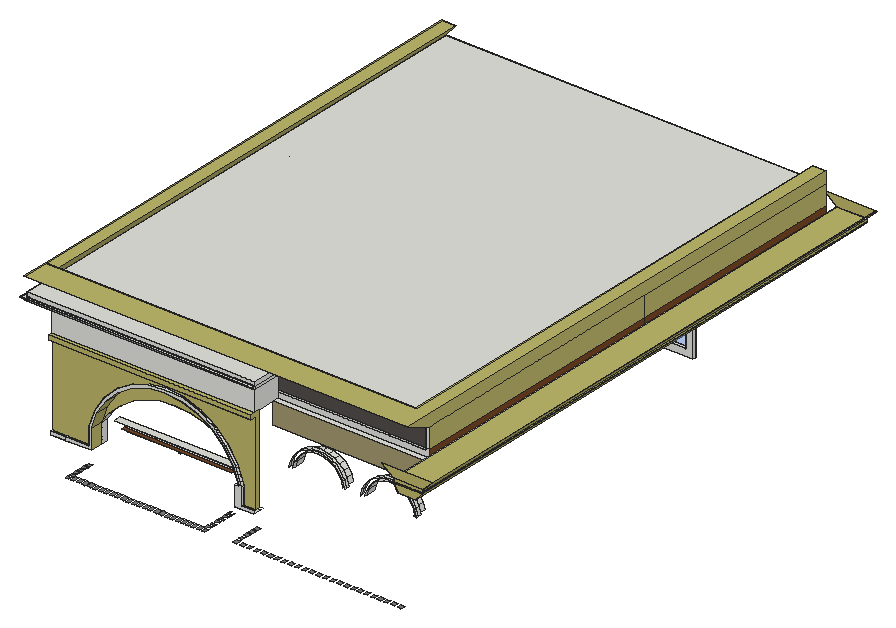
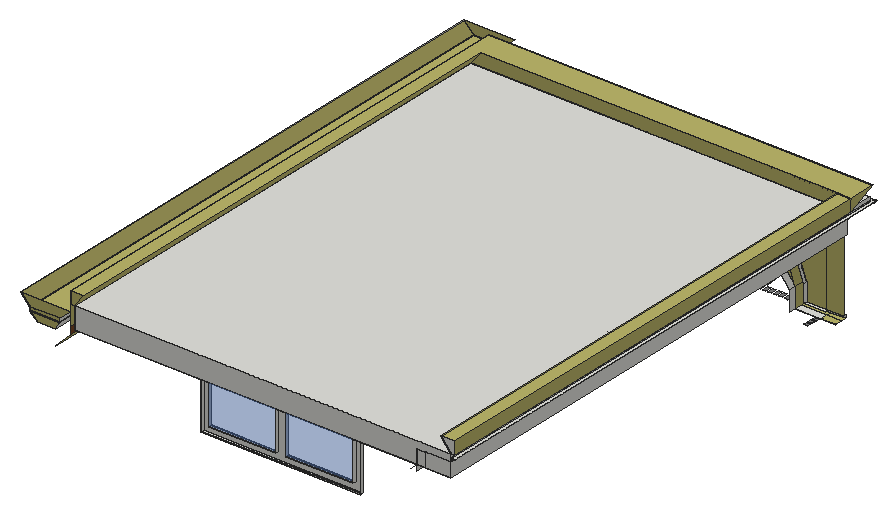
# SketchUp Ruby script. Lengths in inches.
U = 1.inch
M = Sketchup.active_model
def pt(a) = Geom::Point3d.new(a.map { |v| v * U })
def face(e, loops, mat)
  f = e.add_face(loops[0].map { |a| pt(a) })
  loops[1..].each { |l| e.add_face(l.map { |a| pt(a) }).erase! }
  f.material = f.back_material = mat if mat
  f
end
# faces: each face lists its corners as indices into pts; further lists are holes
def faces(e, pts, list, mat = nil) = list.each { |f| face(e, (f[0].is_a?(Array) ? f : [f]).map { |l| l.map { |i| pts[i] } }, mat) }
# xy, xz, yz: faces in a plane at the given z, y or x. An outline is a flat list of corners, or four numbers for a rectangle; further outlines are holes
def ring(l) = l.size == 4 ? [[l[0], l[1]], [l[2], l[1]], [l[2], l[3]], [l[0], l[3]]] : l.each_slice(2).to_a
def flat(e, list, mat, &to3) = list.each { |f| face(e, (f[0].is_a?(Array) ? f : [f]).map { |l| ring(l).map { |u, v| to3.(u, v) } }, mat) }
def xy(e, z, list, mat = nil) = flat(e, list, mat) { |x, y| [x, y, z] }
def xz(e, y, list, mat = nil) = flat(e, list, mat) { |x, z| [x, y, z] }
def yz(e, x, list, mat = nil) = flat(e, list, mat) { |y, z| [x, y, z] }
def lines(e, pts, list) = list.each { |a, b| e.add_line(pt(pts[a]), pt(pts[b])) }
# prism: a flat outline (further loops are holes) pulled along v
def prism(e, loops, v, mat = nil)
  f = face(e, loops, mat); d = Geom::Vector3d.new(v.map { |x| x * U })
  f.pushpull(f.normal.samedirection?(d) ? d.length : -d.length)
end
def box(e, o, s, mat = nil) = prism(e, [[o, [o[0] + s[0], o[1], o[2]], [o[0] + s[0], o[1] + s[1], o[2]], [o[0], o[1] + s[1], o[2]]]], [0, 0, s[2]], mat)
def at(x, y, z, deg = 0) = Geom::Transformation.translation(pt([x, y, z])) * Geom::Transformation.rotation(ORIGIN, Z_AXIS, deg.degrees)
def axes(o, x, y, z) = Geom::Transformation.new([*x, 0, *y, 0, *z, 0, *pt(o).to_a, 1])
def part(name) = M.definitions.add(name)
# library, detail: a bought-in or finely detailed component or shape, given as its bounding box
def library(name, o, s) = part(name).tap { |d| box(d.entities, o, s) }
def detail(e, o, s) = box(e.add_group.entities, o, s)
def put(e, d, t, mat = nil) = e.add_instance(d, t).tap { |i| i.material = mat if mat }
def group(e, t, mat = nil) = e.add_group.tap { |g| g.transformation = t; g.material = mat if mat }.entities
root = M.entities
M.materials.add("[0057_DarkKhaki]").color = [189, 183, 107]
M.materials.add("[0133_Gray]").color = [128, 128, 128]
M.materials.add("[Roofing Shingles GAF Estates]").color = [81, 77, 74]
M.materials.add("[Translucent Glass Blue]").color = [100, 149, 237]
M.materials["[Translucent Glass Blue]"].alpha = 0.5
M.materials.add("[Wood Lumber ButtJoined]").color = [164, 152, 112]
M.materials.add("[Wood Veneer 01]").color = [120, 70, 37]
xy(root,170.03,[[166.125,507.5,323.3,510.5]])
xy(root,170.16,[[194.57,96.25,199.44,96.5625]])
xy(root,170.16,[[61.7,59.0625,64.79,62.04],[67.14,59.0625,70.22,65.0625],[72.57,59.0625,75.66,65.0625],[78.01,59.0625,81.1,65.0625],[83.45,59.0625,86.54,65.0625],
  [88.89,59.0625,91.97,65.0625],[94.32,59.0625,97.41,65.0625],[99.76,59.0625,102.85,65.0625],[105.2,59.0625,108.29,65.0625],[110.64,59.0625,113.72,65.0625],
  [116.07,59.0625,119.16,65.0625],[121.51,59.0625,124.6,65.0625],[126.95,59.0625,130.04,65.0625],[132.39,59.0625,135.47,65.0625],[137.82,59.0625,140.91,65.0625],
  [143.26,59.0625,146.35,65.0625],[148.7,59.0625,151.79,65.0625],[154.14,59.0625,157.22,65.0625],[159.57,59.0625,162.66,65.0625],[165.01,59.0625,168.1,65.0625],
  [170.45,59.0625,173.54,65.0625],[175.64,59.0625,178.72,65.0625],[180.82,59.0625,183.91,65.0625],[186.01,59.0625,189.1,65.0625],[191.2,59.0625,194.29,65.0625],
  [196.39,59.0625,199.44,64.52],[226.06,60.1875,229.86,60.1875,229.86,64.21,229.2,64.21,229.2,65.875,226.06,65.875],[232.93,60.1875,236.73,64.21],[239.81,60.1875,243.61,64.21],[246.68,60.1875,250.48,64.21],
  [253.56,60.1875,257.36,64.21],[260.43,60.1875,264.23,64.21],[267.31,60.1875,271.11,64.21],[274.18,60.1875,277.98,64.21],[281.06,60.1875,284.86,64.21],
  [287.93,60.1875,291.73,64.21],[294.81,60.1875,298.61,64.21],[301.68,60.1875,305.48,64.21],[308.56,60.1875,312.36,64.21],[315.43,60.1875,319.23,64.21],
  [322.31,60.1875,326.11,64.21],[329.18,60.1875,332.98,64.21],[336.06,60.1875,339.86,64.21],[342.68,60.1875,346.48,64.21],[349.31,60.1875,353.11,64.21],
  [355.93,60.1875,359.73,64.21],[362.56,60.1875,366.36,64.21],[369.18,60.1875,372.98,64.21],[375.81,60.1875,379.61,64.21],[382.43,60.1875,386.23,64.21],
  [389.06,60.1875,392.86,64.21],[61.7,64.125,64.79,64.125,64.79,65.0625,65.84,65.0625,65.84,67.1,61.7,67.1],[194.57,65.0625,196.39,65.0625,196.39,67.1875,199.44,67.1875,199.44,69.52,194.57,69.52],[226.06,68.17,229.2,72.0625],[61.7,69.1875,65.84,72.16],
  [194.57,72.1875,199.44,74.52],[61.7,74.25,65.84,77.22],[226.06,74.35,229.2,78.25],[194.57,77.1875,199.44,79.52],[61.7,79.3125,65.84,82.29],
  [226.06,80.54,229.2,84.4375],[194.57,82.1875,199.44,84.52],[61.7,84.375,65.84,87.625],[226.06,86.73,229.2,90.625],[194.57,87.1875,199.44,89.52],
  [194.57,92.1875,199.44,93.58]],"[0133_Gray]")
xy(root,177.07,[[173.17,507.5,239.9,510.5],[249.77,507.5,316.26,510.5]])
xy(root,186.28,[[210.07,82.875,229.2,90.625],[43.3125,87.625,68.39,94.9375],[28.5625,94.9375,43.3125,95.4375],[43.3125,94.9375,68.39,95.4375]])
xy(root,186.28,[[28.5625,82.875,43.3125,87.625],[43.3125,82.875,68.39,87.625],[28.5625,87.625,43.3125,94.9375]],"[0057_DarkKhaki]")
xy(root,189.28,[[28.5625,82.875,43.3125,85.1875],[43.3125,82.875,65.39,85.1875],[217.14,82.875,229.2,85.1875],[43.3125,85.1875,65.39,88.1875],[217.14,85.1875,229.2,88.1875]])
xy(root,202.75,[[141.78,100.3125,143.625,102.3125]])
xy(root,202.75,[[141.78,99.3125,143.625,100.3125],[90.22,100.3125,141.78,102.3125],[143.625,100.3125,193.35,102.3125]],"[Wood Veneer 01]")
xy(root,205.75,[[87.22,100.3125,196.35,102.3125]])
xy(root,205.75,[[87.22,96.3125,196.35,100.3125]],"[Wood Veneer 01]")
xy(root,205.78,[[210.07,82.875,214.14,95.25],[210.07,95.25,214.14,102.3125]])
xy(root,211.67,[[81.29,96.3125,202.27,102.3125]])
xy(root,211.75,[[81.22,95.25,202.35,102.3125]])
xy(root,218.72,[[363.56,112.125,366.56,113.875]])
xy(root,252.6,[[173.17,507.5,239.9,510.5],[249.77,507.5,316.26,510.5]])
xy(root,255,[[229.2,106.125,379.33,112.125]])
xy(root,259.64,[[166.125,507.5,323.3,510.5]])
xy(root,271.48,[[28.5625,79.4375,229.2,85.1875]])
xy(root,276,[[394.3125,54.1875,406.875,54.1875,406.875,550.125,411.75,550.125,411.75,601.9375,394.3125,601.9375],[406.875,54.1875,411.75,550.125],[229.2,106.125,379.33,112.125],[229.2,112.125,379.41,116.875],[379.41,112.125,379.66,116.875],
  [379.41,116.875,379.66,376.8125],[37.25,376.8125,43.3125,510.5],[43.3125,510.5,379.41,550.125]])
xy(root,276,[[28.5625,79.4375,229.2,83.625]],"[0057_DarkKhaki]")
xy(root,281.9375,[[3.4375,112.125,375.74,601.9375]],"[Wood Veneer 01]")
xy(root,283.41,[[390.09,54.1875,419.28,601.9375]])
xy(root,284.03,[[390.09,54.1875,419.28,601.9375]])
xy(root,287.16,[[390.09,54.1875,419.28,601.9375]],"[0057_DarkKhaki]")
xy(root,295.8125,[[3.4375,83.625,28.5625,601.9375]])
xy(root,298.9375,[[0,80.5,0,601.9375,3.4375,601.9375,3.4375,83.625,229.2,83.625,229.2,80.5]])
xy(root,299.125,[[0,80.5,229.2,80.5,229.2,83.625,3.4375,83.625,3.4375,601.9375,0,601.9375]])
xy(root,303.3125,[[3.4375,83.625,229.2,112.125],[0,112.125,3.4375,601.9375],[3.4375,112.125,375.74,601.9375],[375.74,112.125,379.66,112.125,379.66,376.8125,379.41,376.8125,379.41,601.9375,375.74,601.9375],[379.41,376.8125,379.66,601.9375]])
xy(root,315.25,[[0,85.375,379.66,85.375,379.66,601.9375,366.13,601.9375,366.13,112.125,0,112.125],[0,112.125,13.17,601.9375]],"[0057_DarkKhaki]")
xz(root,54.1875,[[390.09,283.41,419.28,284.03],[419.73,286.73,429.15,296.57,428.69,297.01,419.28,287.16]])
xz(root,54.1875,[[394.3125,276,411.75,276,419.28,283.41,390.09,283.41],[390.09,284.03,419.28,287.16],[390.09,287.16,419.28,287.16,428.69,297.01,378.88,297.01]],"[0057_DarkKhaki]")
xz(root,79.4375,[[28.5625,271.48,229.2,276]],"[0057_DarkKhaki]")
xz(root,80.5,[[0,298.9375,3.4375,299.125],[3.4375,298.9375,229.2,299.125]])
xz(root,82.875,[[28.5625,186.28,43.3125,189.28],[43.3125,186.28,68.39,186.28,68.39,205.78,74.12,221.34,83.13,235.27,94.98,246.875,109.09,255.6,124.78,261.01,141.26,262.84,157.75,261.01,173.43,255.6,187.54,246.875,199.39,235.27,208.4,221.34,214.14,205.78,210.07,205.78,210.07,186.28,229.2,186.28,229.2,189.28,217.14,189.28,217.14,206.3125,211.1,222.69,201.73,237.18,189.4,249.25,174.72,258.33,158.41,263.95,141.26,265.86,124.11,263.95,107.8,258.33,93.12,249.25,80.8,237.18,71.42,222.69,65.39,206.3125,65.39,189.28,43.3125,189.28]])
xz(root,83.625,[[28.5625,276,229.2,295.8125],[3.4375,295.8125,229.2,295.8125,225.875,298.9375,3.4375,298.9375],[229.2,295.8125,229.2,298.9375,225.875,298.9375],[3.4375,298.9375,229.2,299.125],[3.4375,299.125,229.2,303.3125]])
xz(root,85.1875,[[28.5625,189.28,65.39,189.28,65.39,206.3125,71.42,222.69,80.8,237.18,93.12,249.25,107.8,258.33,124.11,263.95,141.26,265.86,158.41,263.95,174.72,258.33,189.4,249.25,201.73,237.18,211.1,222.69,217.14,206.3125,217.14,189.28,229.2,189.28,229.2,271.48,28.5625,271.48]],"[0057_DarkKhaki]")
xz(root,95.25,[[68.39,205.78,77.07,217.36,87.58,227.33,99.61,235.38,112.82,241.31,126.83,244.93,141.26,246.15,155.6875,244.93,169.71,241.31,182.92,235.38,194.95,227.33,205.45,217.36,214.14,205.78,208.4,221.34,199.39,235.27,187.54,246.875,173.43,255.6,157.75,261.01,141.26,262.84,124.78,261.01,109.09,255.6,94.98,246.875,83.13,235.27,74.12,221.34]],"[0057_DarkKhaki]")
xz(root,106.125,[[229.2,255,379.33,276]],"[Wood Lumber ButtJoined]")
xz(root,112.125,[[229.2,276,379.41,276,379.66,276.25,379.66,283.8125,375.74,283.8125,375.74,281.9375,229.2,281.9375],[379.41,276,379.66,276,379.66,276.25],[3.4375,281.9375,229.2,303.3125],[229.2,281.9375,375.74,283.8125],[375.74,283.8125,379.66,303.3125],
  [0,303.3125,3.4375,303.3125,13.17,315.25,0,315.25]])
xz(root,112.125,[[3.4375,303.3125,13.17,315.25,366.13,315.25,375.74,303.3125]],"[0057_DarkKhaki]")
xz(root,112.125,[[229.2,283.8125,375.74,303.3125]],"[Roofing Shingles GAF Estates]")
xz(root,116.875,[[391.71,258.49,376.8,273.39,379.41,276,394.3125,261.1]])
xz(root,376.8125,[[391.71,258.49,376.8,273.39,378.97,275.56,393.87,260.66],[379.41,276,379.41,283.8125,379.66,283.8125,379.66,276.25],[379.41,276,379.66,276,379.66,276.25],[379.41,283.8125,379.66,303.3125]])
xz(root,507.5,[[[166.125,170.03,323.3,259.64],[173.17,177.07,239.9,252.6],[249.77,177.07,316.26,252.6]]])
xz(root,510.5,[[[165.9,169.8,323.53,259.87],[166.125,170.03,323.3,259.64]]])
xz(root,510.5,[[173.17,177.07,239.9,252.6],[249.77,177.07,316.26,252.6]],"[Translucent Glass Blue]")
xz(root,601.9375,[[3.4375,281.9375,28.5625,295.8125],[37.25,281.9375,37.25,295.8125,3.4375,295.8125,3.4375,303.3125,375.74,303.3125,375.74,281.9375],[28.5625,281.9375,37.25,295.8125],[390.09,283.41,419.28,284.03],[419.73,286.73,419.28,287.16,428.69,297.01,429.15,296.57],
  [3.4375,295.8125,0.19,298.9375,3.4375,298.9375],[379.41,296.54,378.88,297.01,379.41,297.01],[0,298.9375,3.4375,299.125],[0,303.3125,0,315.25,13.17,315.25,3.4375,303.3125]])
xz(root,601.9375,[[394.3125,276,390.09,283.41,419.28,283.41,411.75,276],[390.09,284.03,419.28,287.16],[390.09,287.16,379.41,296.54,379.41,297.01,428.69,297.01,419.28,287.16],[375.74,303.3125,366.13,315.25,379.66,315.25,379.66,303.3125]],"[0057_DarkKhaki]")
yz(root,0,[[80.5,298.9375,83.625,299.125],[83.625,298.9375,601.9375,299.125]])
yz(root,0,[[112.125,303.3125,85.375,315.25,112.125,315.25],[112.125,303.3125,601.9375,315.25]],"[0057_DarkKhaki]")
yz(root,3.4375,[[112.125,281.9375,601.9375,295.8125],[83.625,295.8125,112.125,298.9375],[112.125,295.8125,601.9375,298.9375],[83.625,298.9375,112.125,299.125],[112.125,298.9375,601.9375,299.125],
  [83.625,299.125,112.125,303.3125],[112.125,299.125,601.9375,303.3125]])
yz(root,37.25,[[376.8125,276,601.9375,295.8125]])
yz(root,65.39,[[82.875,189.28,85.1875,206.3125],[85.1875,189.28,88.1875,206.3125]])
yz(root,68.39,[[95.25,186.28,102.3125,205.78]])
yz(root,68.39,[[82.875,186.28,95.25,205.78]],"[0057_DarkKhaki]")
yz(root,166.125,[[507.5,170.03,510.5,259.64]])
yz(root,173.17,[[507.5,177.07,510.5,252.6]])
yz(root,217.14,[[82.875,189.28,85.1875,206.3125],[85.1875,189.28,88.1875,206.3125]])
yz(root,229.2,[[83.625,276,112.125,295.8125],[112.125,276,116.875,283.8125],[83.625,295.8125,83.625,298.9375,80.68,298.9375],[83.625,295.8125,112.125,298.9375],[80.5,298.9375,80.68,298.9375,80.5,299.125],
  [80.68,298.9375,83.625,298.9375,83.625,299.125,80.5,299.125],[83.625,298.9375,112.125,303.3125]])
yz(root,229.2,[[85.1875,189.28,88.1875,189.28,88.1875,276,79.4375,276,79.4375,271.48,85.1875,271.48]],"[0057_DarkKhaki]")
yz(root,239.9,[[507.5,177.07,510.5,252.6]])
yz(root,249.77,[[507.5,177.07,510.5,252.6]])
yz(root,316.26,[[507.5,177.07,510.5,252.6]])
yz(root,323.3,[[507.5,170.03,510.5,259.64]])
yz(root,375.74,[[112.125,281.9375,601.9375,303.3125]])
yz(root,379.33,[[106.125,255,112.125,276]])
yz(root,379.41,[[376.8125,283.8125,601.9375,303.3125]],"[0057_DarkKhaki]")
yz(root,379.41,[[376.8125,276,601.9375,283.8125]],"[Wood Veneer 01]")
yz(root,379.66,[[112.125,276,376.8125,276.25]])
yz(root,379.66,[[112.125,283.8125,376.8125,303.3125],[112.125,303.3125,601.9375,303.3125,601.9375,315.25,85.375,315.25]],"[0057_DarkKhaki]")
yz(root,379.66,[[112.125,276.25,376.8125,283.8125]],"[Wood Veneer 01]")
yz(root,390.09,[[54.1875,283.41,601.9375,284.03],[54.1875,284.03,601.9375,287.16]])
yz(root,419.28,[[54.1875,283.41,601.9375,284.03]])
yz(root,419.28,[[54.1875,284.03,601.9375,287.16]],"[0057_DarkKhaki]")
p = [[68.39,82.875,205.78],[68.39,95.25,205.78],[74.12,95.25,221.34],[74.12,82.875,221.34],[208.4,82.875,221.34],[208.4,95.25,221.34],
  [214.14,95.25,205.78],[214.14,82.875,205.78],[68.39,102.3125,205.78],[77.07,102.3125,217.36],[77.07,95.25,217.36],[205.45,102.3125,217.36],
  [214.14,102.3125,205.78],[205.45,95.25,217.36],[71.42,85.1875,222.69],[65.39,85.1875,206.3125],[65.39,82.875,206.3125],[71.42,82.875,222.69],
  [217.14,85.1875,206.3125],[211.1,85.1875,222.69],[211.1,82.875,222.69],[217.14,82.875,206.3125],[71.42,88.1875,222.69],[65.39,88.1875,206.3125],
  [217.14,88.1875,206.3125],[211.1,88.1875,222.69],[87.58,102.3125,227.33],[87.58,95.25,227.33],[194.95,102.3125,227.33],[194.95,95.25,227.33],
  [242.99,116.875,218.3125],[244.57,116.875,224.01],[244.57,113.875,224.01],[242.99,113.875,218.3125],[290.98,116.875,224.01],[292.56,116.875,218.3125],
  [292.56,113.875,218.3125],[290.98,113.875,224.01],[313.99,116.875,218.3125],[315.57,116.875,224.01],[315.57,113.875,224.01],[313.99,113.875,218.3125],
  [361.98,116.875,224.01],[363.56,116.875,218.3125],[363.56,113.875,218.3125],[361.98,113.875,224.01],[242.99,125.875,218.3125],[244.57,125.875,224.01],
  [290.98,125.875,224.01],[292.56,125.875,218.3125],[313.99,125.875,218.3125],[315.57,125.875,224.01],[361.98,125.875,224.01],[363.56,125.875,218.3125],
  [239.99,112.125,218.72],[239.99,113.875,218.72],[241.77,113.875,225.16],[241.77,112.125,225.16],[293.77,112.125,225.16],[293.77,113.875,225.16],
  [295.56,113.875,218.72],[295.56,112.125,218.72],[310.99,112.125,218.72],[310.99,113.875,218.72],[312.77,113.875,225.16],[312.77,112.125,225.16],
  [364.77,112.125,225.16],[364.77,113.875,225.16],[366.56,113.875,218.72],[366.56,112.125,218.72],[239.99,116.875,218.72],[241.77,116.875,225.16],
  [293.77,116.875,225.16],[295.56,116.875,218.72],[310.99,116.875,218.72],[312.77,116.875,225.16],[364.77,116.875,225.16],[366.56,116.875,218.72],
  [83.13,95.25,235.27],[83.13,82.875,235.27],[199.39,82.875,235.27],[199.39,95.25,235.27],[80.8,85.1875,237.18],[80.8,82.875,237.18],
  [201.73,85.1875,237.18],[201.73,82.875,237.18],[80.8,88.1875,237.18],[201.73,88.1875,237.18],[247.44,116.875,229.1875],[247.44,113.875,229.1875],
  [288.11,116.875,229.1875],[288.11,113.875,229.1875],[318.44,116.875,229.1875],[318.44,113.875,229.1875],[359.11,116.875,229.1875],[359.11,113.875,229.1875],
  [247.44,125.875,229.1875],[288.11,125.875,229.1875],[318.44,125.875,229.1875],[359.11,125.875,229.1875],[244.99,113.875,230.95],[244.99,112.125,230.95],
  [290.56,112.125,230.95],[290.56,113.875,230.95],[315.99,113.875,230.95],[315.99,112.125,230.95],[361.56,112.125,230.95],[361.56,113.875,230.95],
  [244.99,116.875,230.95],[290.56,116.875,230.95],[315.99,116.875,230.95],[361.56,116.875,230.95],[99.61,102.3125,235.38],[99.61,95.25,235.38],
  [182.92,102.3125,235.38],[182.92,95.25,235.38],[251.44,116.875,233.54],[251.44,113.875,233.54],[284.11,116.875,233.54],[284.11,113.875,233.54],
  [322.44,116.875,233.54],[322.44,113.875,233.54],[355.11,116.875,233.54],[355.11,113.875,233.54],[251.44,125.875,233.54],[284.11,125.875,233.54],
  [322.44,125.875,233.54],[355.11,125.875,233.54],[249.47,113.875,235.84],[249.47,112.125,235.84],[286.08,112.125,235.84],[286.08,113.875,235.84],
  [320.47,113.875,235.84],[320.47,112.125,235.84],[357.08,112.125,235.84],[357.08,113.875,235.84],[249.47,116.875,235.84],[286.08,116.875,235.84],
  [320.47,116.875,235.84],[357.08,116.875,235.84],[256.35,116.875,236.84],[256.35,113.875,236.84],[279.2,116.875,236.84],[279.2,113.875,236.84],
  [327.35,116.875,236.84],[327.35,113.875,236.84],[350.2,116.875,236.84],[350.2,113.875,236.84],[256.35,125.875,236.84],[279.2,125.875,236.84],
  [327.35,125.875,236.84],[350.2,125.875,236.84],[94.98,95.25,246.875],[94.98,82.875,246.875],[187.54,82.875,246.875],[187.54,95.25,246.875],
  [112.82,102.3125,241.31],[112.82,95.25,241.31],[169.71,102.3125,241.31],[169.71,95.25,241.31],[254.98,113.875,239.53],[254.98,112.125,239.53],
  [280.57,112.125,239.53],[280.57,113.875,239.53],[325.98,113.875,239.53],[325.98,112.125,239.53],[351.57,112.125,239.53],[351.57,113.875,239.53],
  [254.98,116.875,239.53],[280.57,116.875,239.53],[325.98,116.875,239.53],[351.57,116.875,239.53],[261.9,116.875,238.9],[261.9,113.875,238.9],
  [273.65,116.875,238.9],[273.65,113.875,238.9],[332.9,116.875,238.9],[332.9,113.875,238.9],[344.65,116.875,238.9],[344.65,113.875,238.9],
  [261.9,125.875,238.9],[273.65,125.875,238.9],[332.9,125.875,238.9],[344.65,125.875,238.9],[93.12,85.1875,249.25],[93.12,82.875,249.25],
  [189.4,85.1875,249.25],[189.4,82.875,249.25],[93.12,88.1875,249.25],[189.4,88.1875,249.25],[267.77,116.875,239.59],[267.77,113.875,239.59],
  [338.77,116.875,239.59],[338.77,113.875,239.59],[267.77,125.875,239.59],[338.77,125.875,239.59],[261.19,113.875,241.83],[261.19,112.125,241.83],
  [274.36,112.125,241.83],[274.36,113.875,241.83],[332.19,113.875,241.83],[332.19,112.125,241.83],[345.36,112.125,241.83],[345.36,113.875,241.83],
  [261.19,116.875,241.83],[274.36,116.875,241.83],[332.19,116.875,241.83],[345.36,116.875,241.83],[126.83,102.3125,244.93],[126.83,95.25,244.93],
  [155.6875,102.3125,244.93],[155.6875,95.25,244.93],[267.77,113.875,242.62],[267.77,112.125,242.62],[338.77,113.875,242.62],[338.77,112.125,242.62],
  [267.77,116.875,242.62],[338.77,116.875,242.62],[141.26,102.3125,246.15],[141.26,95.25,246.15],[109.09,95.25,255.6],[109.09,82.875,255.6],
  [173.43,82.875,255.6],[173.43,95.25,255.6],[107.8,85.1875,258.33],[107.8,82.875,258.33],[174.72,85.1875,258.33],[174.72,82.875,258.33],
  [107.8,88.1875,258.33],[174.72,88.1875,258.33],[124.78,95.25,261.01],[124.78,82.875,261.01],[157.75,82.875,261.01],[157.75,95.25,261.01],
  [124.11,85.1875,263.95],[124.11,82.875,263.95],[158.41,85.1875,263.95],[158.41,82.875,263.95],[124.11,88.1875,263.95],[158.41,88.1875,263.95],
  [376.8,116.875,273.39],[376.8,376.8125,273.39],[391.71,376.8125,258.49],[391.71,367.8125,258.49],[391.71,125.875,258.49],[391.71,116.875,258.49],
  [394.3125,125.875,261.1],[394.3125,116.875,261.1],[394.3125,367.8125,261.1],[394.3125,376.8125,261.1],[393.87,376.8125,260.66],[378.97,376.8125,275.56],
  [378.97,510.5,275.56],[393.87,510.5,260.66],[394.3125,510.5,261.1],[141.26,95.25,262.84],[141.26,82.875,262.84],[379.41,116.875,276],
  [379.41,112.125,276],[394.3125,112.125,261.1],[394.3125,601.9375,261.1],[379.41,601.9375,276],[379.41,550.125,276],[379.41,510.5,276],
  [379.41,376.8125,276],[396.65,367.8125,263.4375],[396.65,125.875,263.4375],[396.65,376.8125,263.4375],[395.5625,510.5,262.35],[398.2,510.5,264.99],
  [398.2,376.8125,264.99],[141.26,85.1875,265.86],[141.26,82.875,265.86],[141.26,88.1875,265.86],[394.3125,54.1875,276],[390.09,54.1875,283.41],
  [390.09,601.9375,283.41],[394.3125,601.9375,276],[419.28,54.1875,283.41],[411.75,54.1875,276],[411.75,550.125,276],[411.75,601.9375,276],
  [419.28,601.9375,283.41],[379.66,112.125,276.25],[379.66,376.8125,276.25],[419.28,54.1875,287.16],[419.28,601.9375,287.16],[419.73,601.9375,286.73],
  [419.73,54.1875,286.73],[429.15,54.1875,296.57],[429.15,601.9375,296.57],[428.69,54.1875,297.01],[428.69,601.9375,297.01],[3.4375,83.625,295.8125],
  [0,80.5,299.125],[0,83.625,299.125],[3.4375,80.5,299.125],[28.5625,83.625,295.8125],[229.2,83.625,295.8125],[229.2,80.68,298.9375],
  [229.2,80.5,299.125],[379.66,112.125,303.3125],[379.66,85.375,315.25],[0,85.375,315.25],[0,112.125,303.3125],[3.4375,112.125,303.3125],
  [229.2,112.125,303.3125],[375.74,112.125,303.3125],[13.17,112.125,315.25],[3.4375,601.9375,303.3125],[13.17,601.9375,315.25],[366.13,112.125,315.25],
  [366.13,601.9375,315.25],[375.74,601.9375,303.3125],[43.3125,88.1875,189.28],[43.3125,88.1875,276],[214.14,94.8125,186.28],[229.2,94.8125,186.28],
  [199.44,61.0625,170.16],[199.47,61.0625,170.16],[394.3125,376.8125,268.875],[394.3125,510.5,268.875],[395.5625,510.5,267.625],[394.3125,376.8125,265.78],
  [394.3125,125.875,265.78],[395.5625,510.5,276],[43.3125,550.125,276],[43.3125,601.9375,276],[37.25,510.5,276],[28.5625,510.5,276],
  [28.5625,376.8125,295.8125],[28.5625,376.8125,303.3125]]
faces(root,p,[[0,1,2,3],[4,5,6,7],[3,2,78,79],[80,81,5,4],[79,78,152,153],[154,155,81,80],[153,152,220,221],[222,223,155,154],
  [221,220,230,231],[232,233,223,222],[231,230,255,256],[256,255,233,232],[248,249,254,260,261,262,263,264,257,247,246],[278,279,280,281,282],[289,288,287,290],[285,291,292,286],
  [301,302,303,304,305,306,307],[308,305,309,310],[307,311,312,313]],"[0057_DarkKhaki]")
faces(root,p,[[8,9,10,1],[11,12,6,13],[14,15,16,17],[18,19,20,21],[22,23,15,14],[24,25,19,18],[9,26,27,10],[28,11,13,29],
  [30,31,32,33],[34,35,36,37],[38,39,40,41],[42,43,44,45],[31,30,46,47],[35,34,48,49],[39,38,50,51],[43,42,52,53],
  [54,55,56,57],[58,59,60,61],[62,63,64,65],[66,67,68,69],[70,71,56,55],[72,73,60,59],[74,75,64,63],[76,77,68,67],
  [82,14,17,83],[19,84,85,20],[86,22,14,82],[25,87,84,19],[31,88,89,32],[90,34,37,91],[39,92,93,40],[94,42,45,95],
  [88,31,47,96],[34,90,97,48],[92,39,51,98],[42,94,99,52],[57,56,100,101],[102,103,59,58],[65,64,104,105],[106,107,67,66],
  [71,108,100,56],[109,72,59,103],[75,110,104,64],[111,76,67,107],[26,112,113,27],[114,28,29,115],[88,116,117,89],[118,90,91,119],
  [92,120,121,93],[122,94,95,123],[116,88,96,124],[90,118,125,97],[120,92,98,126],[94,122,127,99],[101,100,128,129],[130,131,103,102],
  [105,104,132,133],[134,135,107,106],[108,136,128,100],[137,109,103,131],[110,138,132,104],[139,111,107,135],[116,140,141,117],[142,118,119,143],
  [120,144,145,121],[146,122,123,147],[140,116,124,148],[118,142,149,125],[144,120,126,150],[122,146,151,127],[112,156,157,113],[158,114,115,159],
  [129,128,160,161],[162,163,131,130],[133,132,164,165],[166,167,135,134],[136,168,160,128],[169,137,131,163],[138,170,164,132],[171,139,135,167],
  [140,172,173,141],[174,142,143,175],[144,176,177,145],[178,146,147,179],[172,140,148,180],[142,174,181,149],[176,144,150,182],[146,178,183,151],
  [184,82,83,185],[84,186,187,85],[188,86,82,184],[87,189,186,84],[172,190,191,173],[190,174,175,191],[176,192,193,177],[192,178,179,193],
  [190,172,180,194],[174,190,194,181],[192,176,182,195],[178,192,195,183],[161,160,196,197],[198,199,163,162],[165,164,200,201],[202,203,167,166],
  [168,204,196,160],[205,169,163,199],[170,206,200,164],[207,171,167,203],[156,208,209,157],[210,158,159,211],[197,196,212,213],[213,212,199,198],
  [201,200,214,215],[215,214,203,202],[204,216,212,196],[216,205,199,212],[206,217,214,200],[217,207,203,214],[208,218,219,209],[218,210,211,219],
  [224,184,185,225],[186,226,227,187],[228,188,184,224],[189,229,226,186],[234,224,225,235],[226,236,237,227],[238,228,224,234],[229,239,236,226],
  [246,247,245,244],[248,246,244,243],[249,248,243,242,250],[254,249,250,253],[247,257,258,259],[246,248,265,266],[248,249,267,265],[249,254,268,269,270,267],
  [271,234,235,272],[236,271,272,237],[273,238,234,271],[239,273,271,236],[257,264,251,241,240],[264,263,252,251],[274,275,276,277],[264,257,258,283,284],
  [285,286,287,288],[293,294,295],[294,293,296],[296,293,297,298,299,300],[292,291,289,290]])
faces(root,p,[[240,241,242,243,244,245],[250,251,252,253]],"[Wood Veneer 01]")
lines(root,p,[[314,315],[316,317],[318,319],[320,270],[321,322],[323,267],[324,266],[322,269],[268,322],[322,325],[326,327],[328,329],
  [330,331]])
